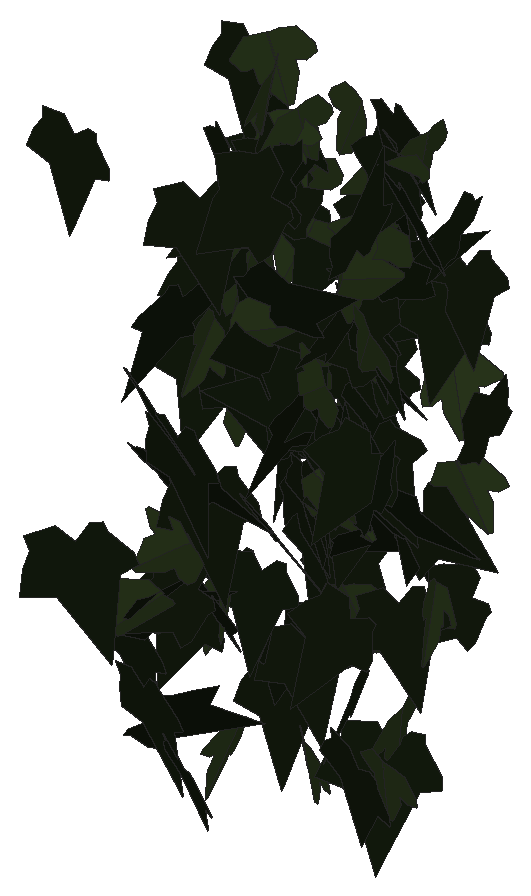
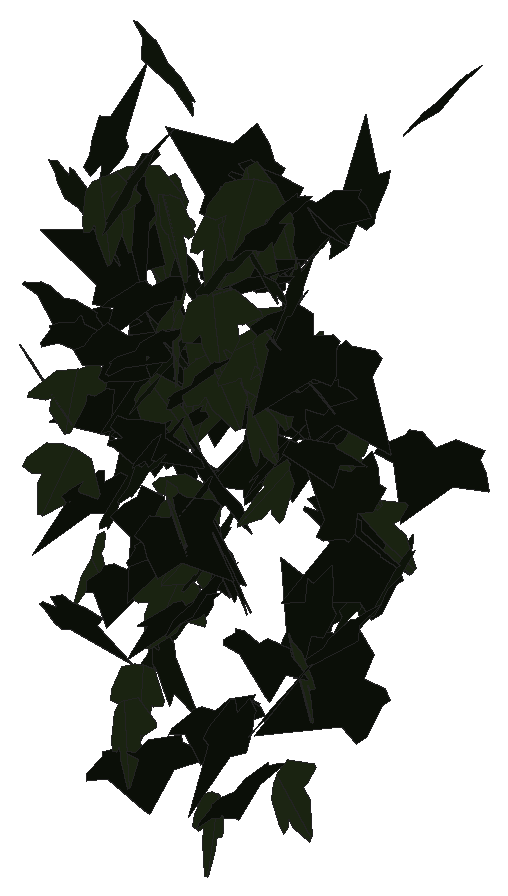
# SketchUp Ruby script. Lengths in inches.
U = 1.inch
M = Sketchup.active_model
def pt(a) = Geom::Point3d.new(a.map { |v| v * U })
def face(e, loops, mat)
  f = e.add_face(loops[0].map { |a| pt(a) })
  loops[1..].each { |l| e.add_face(l.map { |a| pt(a) }).erase! }
  f.material = f.back_material = mat if mat
  f
end
# faces: each face lists its corners as indices into pts; further lists are holes
def faces(e, pts, list, mat = nil) = list.each { |f| face(e, (f[0].is_a?(Array) ? f : [f]).map { |l| l.map { |i| pts[i] } }, mat) }
# xy, xz, yz: faces in a plane at the given z, y or x. An outline is a flat list of corners, or four numbers for a rectangle; further outlines are holes
def ring(l) = l.size == 4 ? [[l[0], l[1]], [l[2], l[1]], [l[2], l[3]], [l[0], l[3]]] : l.each_slice(2).to_a
def flat(e, list, mat, &to3) = list.each { |f| face(e, (f[0].is_a?(Array) ? f : [f]).map { |l| ring(l).map { |u, v| to3.(u, v) } }, mat) }
def xy(e, z, list, mat = nil) = flat(e, list, mat) { |x, y| [x, y, z] }
def xz(e, y, list, mat = nil) = flat(e, list, mat) { |x, z| [x, y, z] }
def yz(e, x, list, mat = nil) = flat(e, list, mat) { |y, z| [x, y, z] }
def lines(e, pts, list) = list.each { |a, b| e.add_line(pt(pts[a]), pt(pts[b])) }
# prism: a flat outline (further loops are holes) pulled along v
def prism(e, loops, v, mat = nil)
  f = face(e, loops, mat); d = Geom::Vector3d.new(v.map { |x| x * U })
  f.pushpull(f.normal.samedirection?(d) ? d.length : -d.length)
end
def box(e, o, s, mat = nil) = prism(e, [[o, [o[0] + s[0], o[1], o[2]], [o[0] + s[0], o[1] + s[1], o[2]], [o[0], o[1] + s[1], o[2]]]], [0, 0, s[2]], mat)
def at(x, y, z, deg = 0) = Geom::Transformation.translation(pt([x, y, z])) * Geom::Transformation.rotation(ORIGIN, Z_AXIS, deg.degrees)
def axes(o, x, y, z) = Geom::Transformation.new([*x, 0, *y, 0, *z, 0, *pt(o).to_a, 1])
def part(name) = M.definitions.add(name)
# library, detail: a bought-in or finely detailed component or shape, given as its bounding box
def library(name, o, s) = part(name).tap { |d| box(d.entities, o, s) }
def detail(e, o, s) = box(e.add_group.entities, o, s)
def put(e, d, t, mat = nil) = e.add_instance(d, t).tap { |i| i.material = mat if mat }
def group(e, t, mat = nil) = e.add_group.tap { |g| g.transformation = t; g.material = mat if mat }.entities
root = M.entities
M.materials.add("efeu1").color = [18, 25, 13]
M.materials.add("efeu2").color = [43, 57, 29]
c1 = part("ivyleaf_9")
p = [[1.54,2.16,1.25],[1.36,2.04,1.19],[-0.21,0.99,0.68],[-0.71,1.11,0.82],[-0.85,0.86,0.67],[-0.8,0.17,0.21],
  [-0.9,-0.01,0.1],[-0.67,-0.16,-0.02],[-0.08,-0.08,-0.05],[-0.03,-0.6,-0.4],[0.65,-0.88,-0.66],[0.83,-0.6,-0.49],
  [1.29,-0.42,-0.43],[1.8125,-0.07,-0.26],[1.21,0.44,0.15]]
faces(c1.entities,p,[[0,1,2,3,4,5,6,7,8,9,10,11,12,13,14]],"efeu1")
c2 = part("ivyleaf_10")
p = [[0,0.5,-0.03],[-0.0625,2.02,-0.43],[-0.19,2.01,-0.46],[-0.54,1.05,-0.29],[-0.52,0.625,-0.18],[-0.83,0.76,-0.28],
  [-1.16,0.64,-0.33],[-1.15,0.33,-0.24],[-0.77,-0.39,0.02],[-0.3,-0.51,0.16],[0.04,-0.48,0.23],[-0.02,2.01,-0.4375],
  [-0.06,2.01,-0.43],[0.04,-0.49,0.23],[0.67,-0.49,0.14],[1.38,0.36,-0.2],[1.375,0.51,-0.24],[0.81,0.65,-0.19],
  [0.62,0.59,-0.15],[0.6,1.09,-0.28],[0.5,1.23,-0.31]]
faces(c2.entities,p,[[0,1,2,3,4,5,6,7,8,9,10],[11,12,0,13,14,15,16,17,18,19,20]],"efeu2")
put(root,c1,axes([598.4375,121.89,296.9375],[0.81397,0.88754,0.23094],[0.14236,0.18276,-1.20414],[-0.90598,0.82612,0.01828]))
put(root,c1,axes([598.96,119.74,294.29],[-0.31391,0.82169,-1.14209],[0.42388,-1.06057,-0.87954],[-1.34159,-0.52735,-0.01066]))
put(root,c1,axes([598.76,121.96,294.49],[-0.45485,-1.05863,-0.34168],[0.17374,0.297,-1.15149],[1.09875,-0.48521,0.04063]))
put(root,c1,axes([598.8,123.95,302.49],[0.01835,-1.25886,0.08215],[-0.04016,-0.0827,-1.25832],[1.2609,0.01569,-0.04128]))
put(root,c1,axes([598.68,123.28,282.36],[0.3209,-1.15031,0.18653],[0.04731,-0.18045,-1.19422],[1.16437,0.32436,-0.00289]))
put(root,c1,axes([598.75,114.04,303.23],[0.04246,-1.24525,0.32852],[0.09612,-0.32472,-1.24326],[1.28426,0.06548,0.08219]))
put(root,c1,axes([598.74,122.83,298.29],[0.05541,-0.69373,1.06934],[0.17581,-1.05596,-0.69416],[1.26248,0.1775,0.04973]))
put(root,c1,axes([600.36,121.47,295.98],[-0.83003,0.81696,0.59511],[-0.47923,0.35991,-1.16247],[-0.8899,-0.95581,0.07094]))
put(root,c1,axes([599.32,121.34,291.92],[-1.00625,-0.86669,-0.42684],[0.50796,0.04963,-1.29823],[0.82179,-1.09191,0.2798]))
put(root,c2,axes([599.65,123.625,296.7],[0.32446,1.12014,-0.30063],[-0.23389,-0.24256,-1.15621],[-1.13595,0.36989,0.15219]))
put(root,c1,axes([599.45,119.72,282.72],[-0.26444,-1.25582,0.57352],[-0.00562,-0.58296,-1.27908],[1.38057,-0.24291,0.10465]))
put(root,c2,axes([599.73,123.33,293.76],[0.31115,-1.07411,0.59459],[0.28911,-0.53204,-1.1124],[1.19318,0.40901,0.11448]))
put(root,c2,axes([600.02,122.11,295.25],[-0.31112,-1.18985,0.25359],[0.00604,-0.26326,-1.2278],[1.21656,-0.30298,0.07095]))
put(root,c2,axes([599.86,123.68,303.125],[-0.88328,-0.85832,-0.26691],[0.32713,0.04158,-1.2163],[0.83722,-0.92179,0.19366]))
put(root,c1,axes([599.02,118.52,288],[0.36773,-0.69134,0.97636],[0.81383,-0.60413,-0.73428],[0.87688,0.85061,0.27204]))
put(root,c2,axes([600.06,120.61,282.5],[0.9123,-0.80986,-0.22247],[-0.13248,0.18559,-1.21888],[0.82935,0.92051,0.05001]))
put(root,c1,axes([600.41,122.71,300.07],[-1.02036,0.27097,-0.61037],[0.55975,-0.26083,-1.05155],[-0.36421,-1.16002,0.09387]))
put(root,c2,axes([600.3,120.96,277.04],[0.25039,-1.1291,0.45866],[0.06524,-0.45515,-1.15608],[1.21695,0.25672,-0.0324]))
put(root,c1,axes([599.79,112.91,287.8125],[-0.57585,-0.84006,-1.0577],[0.56788,0.89268,-1.01817],[1.22554,-0.80837,-0.02519]))
put(root,c2,axes([600.18,121.4,290.1],[0.15432,-0.4838,-1.0836],[0.34432,1.06397,-0.42599],[1.13564,-0.25685,0.27641]))
put(root,c2,axes([600.96,124.41,295.76],[-0.8995,-0.62224,0.52279],[-0.31788,-0.44833,-1.08054],[0.74796,-0.93884,0.1695]))
put(root,c1,axes([599.76,115.82,283.29],[0.57577,-1.259,0.49878],[0.22999,-0.4432,-1.38422],[1.33453,0.61956,0.02336]))
put(root,c1,axes([599.98,121.07,291.74],[0.60134,-1.17618,-0.37828],[-0.07639,0.3845,-1.31698],[1.23315,0.59738,0.10289]))
put(root,c1,axes([600.78,123.25,298.81],[-0.84082,-0.7293,0.5622],[-0.12808,-0.66129,-1.04939],[0.91189,-0.76534,0.37099]))
put(root,c1,axes([600.49,124.27,288.01],[-0.85704,0.08996,-0.83444],[0.82543,-0.1254,-0.8613],[-0.15182,-1.18957,0.02769]))
put(root,c2,axes([601.26,115.19,285.16],[-0.53599,-0.61099,0.90996],[-0.63099,-0.65624,-0.8123],[0.89621,-0.82745,-0.02769]))
put(root,c2,axes([600.6,119.36,293.76],[-0.03018,0.68288,-1.05586],[-0.03607,-1.0562,-0.68206],[-1.25692,0.01391,0.04492]))
put(root,c2,axes([600.86,122.25,302.64],[0.37799,-1.17516,-0.2445],[-0.03448,0.2456,-1.23376],[1.19983,0.37728,0.04157]))
put(root,c2,axes([601.58,119.61,299.1],[-0.61455,0.30427,1.06178],[-1.0199,0.3101,-0.67918],[-0.42399,-1.18697,0.09474]))
put(root,c2,axes([601.1,124.16,298.22],[-0.62964,-1.06262,0.0762],[-0.0324,-0.06937,-1.23513],[1.06485,-0.63043,0.00747]))
put(root,c1,axes([600.55,123.58,277.96],[-0.02078,-1.32132,0.08677],[0.00886,-0.08692,-1.32145],[1.32414,-0.02015,0.0102]))
put(root,c1,axes([600.59,115.36,284.125],[0.76223,0.71598,1.0492],[0.57409,0.89732,-1.02941],[-1.13308,0.93629,0.18424]))
put(root,c1,axes([600.86,121.81,283.17],[-0.86923,-0.51725,-0.66424],[0.58729,0.31152,-1.01113],[0.6032,-1.04868,0.02727]))
put(root,c1,axes([600.44,116.54,279.59],[1.00794,0.72247,0.8533],[0.62983,0.58234,-1.23702],[-0.9238,1.1853,0.08765]))
put(root,c2,axes([600.77,122.76,300.5625],[-1.06964,-0.32937,-0.48835],[0.54446,-0.16648,-1.08025],[0.2248,-1.164,0.29269]))
put(root,c1,axes([600.28,119.58,282.99],[0.155,-0.57797,1.27547],[0.68913,-1.08563,-0.57569],[1.21901,0.68722,0.16327]))
put(root,c1,axes([600.59,124.1,299.9375],[-0.01945,-0.96662,0.79334],[0.36631,-0.76303,-0.92072],[1.19564,0.21805,0.29499]))
put(root,c1,axes([601.21,122.82,280.49],[0.37452,-0.5041,-1.20181],[-0.74587,0.9425,-0.62777],[1.06871,0.83444,-0.01697]))
put(root,c1,axes([601.3,125.1,295.42],[-0.38178,-1.06436,0.43406],[-0.07329,-0.4339,-1.12844],[1.14713,-0.38196,0.07237]))
put(root,c1,axes([601.46,122.17,299.13],[-0.47083,-0.78978,0.87312],[-0.05902,-0.92334,-0.86702],[1.17585,-0.36258,0.3061]))
put(root,c1,axes([601.23,118,299.8],[-0.30507,-1.13496,-0.64938],[0.16607,0.62779,-1.17524],[1.29702,-0.34733,-0.00226]))
put(root,c1,axes([601.92,121.29,297.79],[-1.04047,-0.55378,0.58314],[0.50939,0.28403,1.17862],[-0.62229,1.15843,-0.01022]))
put(root,c1,axes([602.4375,116.11,285.64],[-1.26484,0.12897,0.36633],[-0.36724,0.00895,-1.27111],[-0.12638,-1.3168,0.02724]))
put(root,c2,axes([601.58,123.1,301.05],[-0.34824,-1.12211,-0.3218],[0.23097,0.26294,-1.16682],[1.14426,-0.39458,0.13759]))
put(root,c2,axes([602.51,115.29,287.75],[-0.69998,-0.11219,1.00129],[-0.95587,-0.31155,-0.70313],[0.31857,-1.18131,0.09035]))
put(root,c2,axes([602.3,122.74,276.19],[-0.9735,0.59265,0.33026],[-0.3053,0.13317,-1.13889],[-0.60589,-1.01933,0.04323]))
put(root,c1,axes([601.96,122.47,289.125],[-0.8425,0.83191,0.63268],[0.4259,-0.46884,1.18362],[0.95444,0.94354,0.0303]))
put(root,c1,axes([602.89,124.31,288.79],[-0.14069,0.49418,-1.09361],[-0.59045,-0.98711,-0.37009],[-1.04478,0.49131,0.35643]))
put(root,c1,axes([602.09,122.83,280.42],[-0.19418,-1.12608,-0.4805],[0.12238,0.46621,-1.14206],[1.21818,-0.22634,0.03814]))
put(root,c1,axes([602.4,120.41,293.66],[-0.38373,-0.44349,1.32469],[-0.2637,-1.32607,-0.52033],[1.37185,-0.37895,0.27052]))
put(root,c1,axes([603.17,120.42,300.29],[-1.04679,0.63974,0.05111],[-0.04374,0.02645,-1.2268],[-0.64029,-1.0477,0.00024]))
put(root,c1,axes([601.72,114.35,282.09],[0.65243,-1.21456,0.37859],[0.1989,-0.32286,-1.37853],[1.25655,0.68173,0.02164]))
put(root,c2,axes([602.22,119.2,294.61],[-0.19728,-0.22405,-1.23119],[0.68989,1.02041,-0.29624],[1.04407,-0.71659,-0.0369]))
put(root,c1,axes([603.52,118.8125,300.42],[-1.42936,-0.00754,0.34111],[-0.3411,-0.00369,-1.42937],[0.00819,-1.46949,0.00184]))
put(root,c1,axes([602.26,117.27,289.13],[0.0579,-1.41968,-0.332],[-0.05614,0.32985,-1.42025],[1.4569,0.06913,-0.04153]))
put(root,c2,axes([602.625,124.63,289.625],[0.80806,-0.87014,0.18251],[0.12711,-0.13102,-1.18747],[0.87994,0.81799,0.00394]))
put(root,c2,axes([603.2,124.05,301.49],[0.9832,-0.5553,-0.55425],[-0.352,0.48194,-1.10728],[0.70118,1.02059,0.22131]))
put(root,c2,axes([602.95,122.51,286.98],[-0.08362,-0.32402,-1.17252],[0.2316,1.14955,-0.33418],[1.19421,-0.24563,-0.01729]))
put(root,c1,axes([602.29,122.26,287.04],[-0.23589,-0.21444,-1.17844],[1.17889,0.17097,-0.26709],[0.21195,-1.18959,0.17404]))
put(root,c1,axes([602.48,122.34,290.03],[0.54218,-1.14383,-0.20299],[-0.07477,0.18918,-1.26575],[1.15929,0.54715,0.0133]))
put(root,c1,axes([602.48,122.77,286.75],[0.29937,-1.00836,0.62481],[0.18505,-0.59681,-1.05184],[1.17172,0.35189,0.00648]))
put(root,c1,axes([602.8,123.2,284.91],[-0.02543,-1.18006,0.43503],[-0.0231,-0.4346,-1.18026],[1.25748,-0.03185,-0.01288]))
put(root,c1,axes([602.25,116.08,290.16],[1.07649,-0.25344,0.52385],[0.50702,-0.1322,-1.10586],[0.28563,1.18986,-0.01128]))
put(root,c2,axes([603.75,123.08,295.6],[0.25664,-0.19691,-1.22474],[-0.53921,1.10863,-0.29123],[1.11715,0.58033,0.14079]))
put(root,c1,axes([604.33,119.79,292.15],[-0.52824,-0.12852,1.0872],[-1.05529,-0.26148,-0.54365],[0.29135,-1.18012,0.00205]))
put(root,c2,axes([604.38,123.41,293.08],[-0.80335,0.07999,0.91342],[-0.89077,-0.35606,-0.75224],[0.21743,-1.16316,0.29309]))
put(root,c2,axes([603.67,120.89,292.93],[-0.37571,-1.02996,-0.52044],[0.22167,0.47272,-1.09555],[1.13249,-0.43422,0.04179]))
put(root,c1,axes([604.39,123.25,295.72],[-1.11012,0.34119,-0.34354],[0.30458,-0.1759,-1.15892],[-0.37638,-1.14867,0.07542]))
put(root,c1,axes([604.84,124.55,291.66],[-0.99507,-0.14357,0.67013],[-0.66814,-0.05979,-1.00492],[0.15257,-1.19819,-0.03015]))
put(root,c1,axes([603.61,123.55,291.87],[0.16872,-1.18535,-0.2059],[-0.04226,0.20195,-1.19723],[1.20236,0.17343,-0.01318]))
put(root,c1,axes([603.46,122.98,284.4],[0.37754,-0.93176,-0.6916],[0.09469,0.74959,-0.95821],[1.15651,0.2428,0.30422]))
put(root,c1,axes([603.89,125.14,295.92],[-0.44014,-1.11623,0.28511],[0.00616,-0.30748,-1.19432],[1.15205,-0.42482,0.11531]))
put(root,c1,axes([604.4,119.62,291.86],[-0.4075,0.4158,-1.06374],[0.54744,-0.92012,-0.56937],[-1.00237,-0.67155,0.12149]))
put(root,c2,axes([604.21,122.79,296.32],[-0.17549,1.13497,-0.54632],[0.02762,-0.548,-1.14733],[-1.25931,-0.17018,0.05097]))
put(root,c1,axes([604.29,123.18,287.04],[-0.42409,-1.1442,0.03662],[-0.01087,-0.03502,-1.22027],[1.14474,-0.42423,0.00198]))
put(root,c1,axes([603.7,114.06,279.77],[0.35208,-0.77947,0.88639],[0.4123,-0.7855,-0.85452],[1.10602,0.54095,0.03639]))
put(root,c1,axes([604.01,124.24,298.07],[0.21139,-0.971,-0.71315],[0.11573,0.73707,-0.96926],[1.19918,0.10003,0.21925]))
put(root,c1,axes([603.77,117.9,288.36],[1.02789,-0.57689,0.28594],[0.23723,-0.16143,-1.17847],[0.59857,1.05464,-0.02398]))
put(root,c2,axes([604.1,121.51,288.0625],[-0.90765,-0.13985,-0.81354],[0.82451,-0.09528,-0.90351],[0.0398,-1.21515,0.16447]))
put(root,c2,axes([605.46,119.41,293.29],[-0.65086,0.16423,1.01664],[-1.01986,0.06405,-0.66327],[-0.14286,-1.20543,0.10327]))
put(root,c1,axes([604.12,123.45,294.14],[0.45829,-1.11921,0.29812],[0.13476,-0.2669,-1.20919],[1.15037,0.47715,0.02289]))
put(root,c1,axes([604.42,123.87,290.14],[0.18433,-1.06405,0.72876],[0.27035,-0.68793,-1.07282],[1.26103,0.30302,0.12347]))
put(root,c1,axes([605.875,124.44,294.4],[-0.28658,0.13541,1.18924],[-1.15731,-0.34334,-0.23979],[0.30538,-1.17411,0.20727]))
put(root,c1,axes([604.47,111.6,295.24],[1.21331,-0.69271,-0.54022],[0.51496,-0.18545,1.39436],[-0.7117,-1.31513,0.08793]))
put(root,c2,axes([605.1,121.58,283.9],[-1.1375,-0.24436,-0.30591],[0.29578,0.07954,-1.16336],[0.25653,-1.17523,-0.01513]))
put(root,c1,axes([604.56,122.41,293.25],[1.21035,-0.22878,0.07764],[0.07558,-0.0182,-1.23177],[0.22947,1.2127,-0.00384]))
put(root,c1,axes([606.3125,121.54,294.7],[-0.90459,-0.08563,0.9191],[-0.91705,-0.06342,-0.90849],[0.10529,-1.28802,-0.01637]))
put(root,c1,axes([605.48,121.55,286.71],[0.4566,1.05762,0.23913],[0.11845,0.20927,-1.1517],[-1.07783,0.47103,-0.02526]))
put(root,c1,axes([605.78,121.36,280.94],[-0.79251,0.48977,-0.69106],[0.5812,-0.374,-0.93158],[-0.61616,-0.98273,0.01012]))
put(root,c1,axes([606.17,122.4,300.375],[0.5562,0.02583,-1.1473],[-1.14713,-0.0237,-0.55665],[-0.0326,1.2748,0.0129]))
put(root,c1,axes([605.03,124.08,301.8],[0.73598,-1.00791,0.08638],[0.03474,-0.08157,-1.24786],[1.01101,0.73653,-0.02]))
put(root,c1,axes([606.03,120.33,288.43],[0.74265,-0.34365,0.93272],[-0.38264,0.97574,0.66417],[-0.91742,-0.68515,0.47803]))
put(root,c1,axes([605.69,122.91,277.42],[-0.63172,-1.30854,-0.39119],[0.15684,0.35865,-1.45298],[1.35672,-0.65074,-0.01418]))
put(root,c2,axes([606.1,122.98,278.8],[0.12592,-1.20228,-0.28586],[-0.0094,0.2864,-1.20869],[1.23576,0.12469,0.01993]))
put(root,c1,axes([606.58,119.58,296.49],[-0.91867,0.80914,-0.13427],[0.08821,-0.10297,-1.22405],[-0.81544,-0.92271,0.01886]))
put(root,c2,axes([606.18,124.25,301.19],[-0.08814,-1.25739,-0.08719],[0.00018,0.08739,-1.26047],[1.26041,-0.08795,-0.00592]))
put(root,c2,axes([606.17,122.35,300.86],[-0.75477,-1.00158,-0.09615],[0.08857,0.05359,-1.25354],[1.00227,-0.75898,0.03837]))
put(root,c2,axes([606.52,121.24,298.9375],[-1.08815,-0.46036,0.41268],[-0.32607,-0.28242,-1.17483],[0.52528,-1.12899,0.12561]))
put(root,c1,axes([605.51,122.02,294.6],[0.62148,-1.04,0.1457],[0.09531,-0.11274,-1.21131],[1.04582,0.62829,0.02381]))
put(root,c1,axes([605.48,111.49,294.62],[0.56181,-1.36745,0.26542],[0.10452,-0.244,-1.47836],[1.38904,0.57144,0.00389]))
put(root,c1,axes([606.64,119.375,284.39],[-1.13319,-0.46089,-0.14815],[0.134,0.06373,-1.2233],[0.46519,-1.14106,-0.00849]))
put(root,c1,axes([606.42,122.46,301.03],[-0.15218,-1.04921,0.79209],[-0.02473,-0.79495,-1.05775],[1.31439,-0.13643,0.07181]))
put(root,c1,axes([605.83,116.33,298.11],[0.28091,-0.35415,1.26589],[1.2269,-0.39399,-0.38248],[0.47182,1.23538,0.24091]))
put(root,c2,axes([607.4,117.64,291.04],[-1.04219,0.48543,0.45725],[-0.43573,0.14655,-1.14871],[-0.50484,-1.12861,0.04751]))
put(root,c1,axes([606.4,121.85,297.02],[0.25464,-0.04985,1.34194],[1.29328,0.37684,-0.23141],[-0.36154,1.31288,0.11738]))
put(root,c1,axes([607.89,124.6,283.46],[-1.14139,-0.06918,0.19169],[-0.19301,0.0169,-1.14314],[0.06541,-1.15725,-0.02815]))
put(root,c2,axes([607.18,119.06,298.47],[0.00092,-0.48505,-1.13365],[0.43295,1.0616,-0.45388],[1.15455,-0.3977,0.1711]))
put(root,c1,axes([607.09,121.75,284.08],[-0.20956,-1.09969,-0.5919],[0.16136,0.5713,-1.11855],[1.2384,-0.26052,0.04559]))
put(root,c2,axes([607.82,120.14,278.5],[-1.107,0.21609,0.30852],[-0.29728,0.0869,-1.12757],[-0.2313,-1.1459,-0.02733]))
put(root,c1,axes([607.61,124,295.26],[-0.48862,-1.08793,-0.09546],[0.05148,0.08152,-1.19254],[1.09089,-0.49114,0.01352]))
put(root,c1,axes([607.17,122.04,287.23],[0.18066,-0.8034,1.01493],[0.24493,-0.98504,-0.82334],[1.27104,0.30401,0.0144]))
put(root,c2,axes([608.51,118.41,296.68],[-0.91382,0.26509,0.79226],[-0.75395,0.24408,-0.95131],[-0.35986,-1.18455,-0.01872]))
put(root,c1,axes([607.61,119.55,291.55],[0.04723,-0.99937,-0.91828],[-0.06156,0.91631,-1.0004],[1.3558,0.07642,-0.01343]))
put(root,c2,axes([607.78,123.9375,292.8],[0.58888,1.07279,0.10328],[0.04929,0.09076,-1.22379],[-1.07662,0.59094,0.00046]))
put(root,c1,axes([607.78,122.42,287.74],[0.47121,-0.53052,-1.0117],[-0.24223,1.0231,-0.64932],[1.11639,0.44592,0.28614]))
put(root,c1,axes([607.77,124.64,296.49],[-0.59339,-0.69771,-0.81354],[0.86054,0.24412,-0.83704],[0.63884,-0.97692,0.37186]))
put(root,c2,axes([608.11,122.52,284.45],[-0.14225,0.89512,-0.75729],[0.05337,-0.75711,-0.90493],[-1.17127,-0.14321,0.05073]))
put(root,c1,axes([608.67,118.03,292.27],[-0.9941,-0.72797,-0.00491],[0.00377,0.00316,-1.23214],[0.72797,-0.99411,-0.00033]))
put(root,c2,axes([608.4,123.7,289.02],[-1.06843,-0.33034,-0.38585],[0.41447,-0.04749,-1.10703],[0.29363,-1.13498,0.15862]))
put(root,c1,axes([607.96,118.35,279.35],[0.15144,-1.07001,0.92119],[0.32788,-0.87449,-1.06967],[1.37331,0.32678,0.1538]))
put(root,c1,axes([609.52,121.9375,299.66],[-0.80701,0.93613,0.24763],[-0.19573,0.158,-1.23517],[-0.94834,-0.82923,0.04421]))
put(root,c1,axes([609.5625,117.21,291.05],[-0.03729,0.4332,1.25952],[-0.43347,1.18747,-0.42125],[-1.25942,-0.42153,0.10769]))
put(root,c1,axes([609.06,120.66,300.15],[0.72316,-1.07781,0.32059],[-0.11112,0.3108,1.29555],[-1.11897,-0.72742,0.07853]))
put(root,c1,axes([609.73,116.12,301.89],[-1.04823,0.78346,-0.45317],[-0.36202,0.27258,1.30866],[0.82953,1.10898,-0.00151]))
put(root,c1,axes([608.29,119.32,289.65],[1.1362,-0.15173,0.67227],[0.66178,-0.12169,-1.14593],[0.1924,1.31457,-0.02849]))
put(root,c1,axes([610.1,122.875,291.55],[-0.30264,0.68352,0.93082],[-0.53058,0.77237,-0.73968],[-1.02572,-0.6012,0.10799]))
